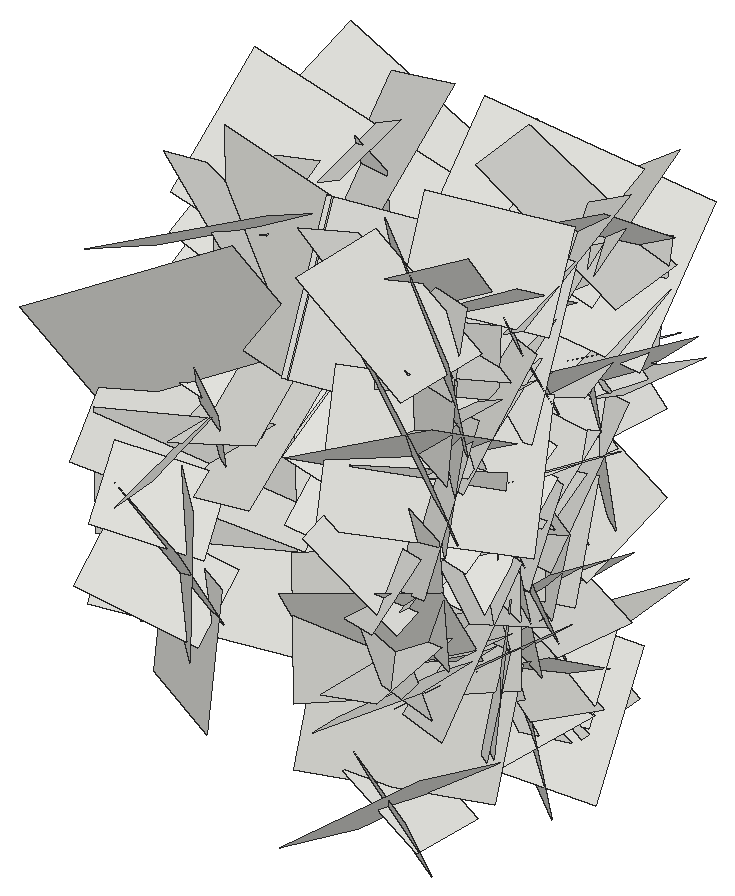
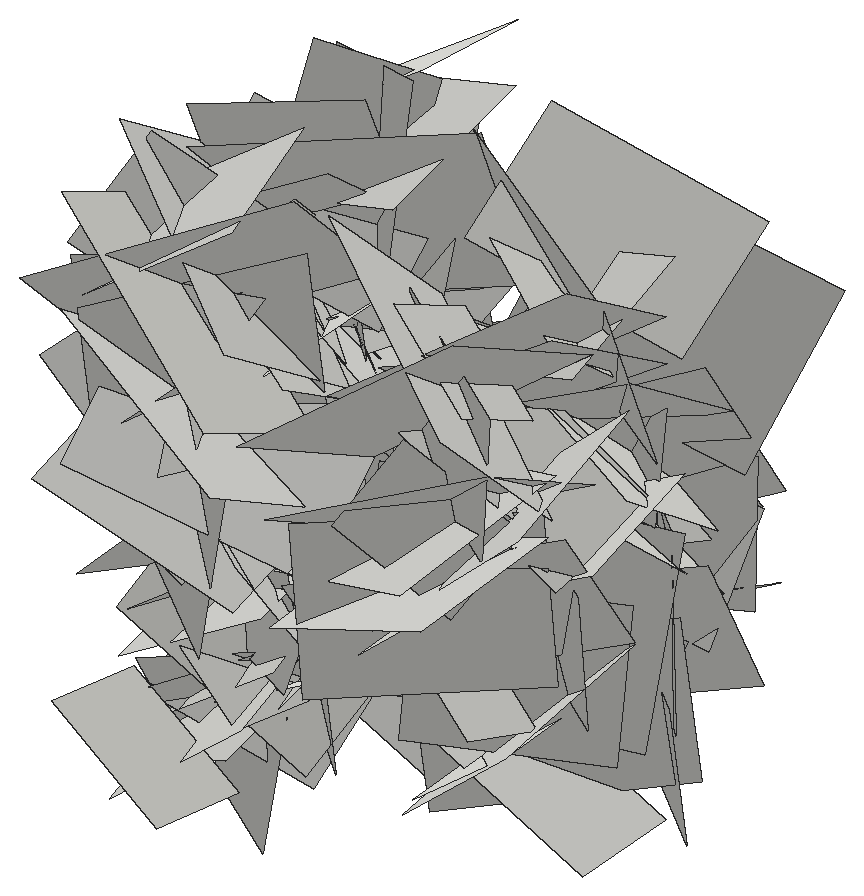
# SketchUp Ruby script. Lengths in inches.
U = 1.inch
M = Sketchup.active_model
def pt(a) = Geom::Point3d.new(a.map { |v| v * U })
def face(e, loops, mat)
  f = e.add_face(loops[0].map { |a| pt(a) })
  loops[1..].each { |l| e.add_face(l.map { |a| pt(a) }).erase! }
  f.material = f.back_material = mat if mat
  f
end
# faces: each face lists its corners as indices into pts; further lists are holes
def faces(e, pts, list, mat = nil) = list.each { |f| face(e, (f[0].is_a?(Array) ? f : [f]).map { |l| l.map { |i| pts[i] } }, mat) }
# xy, xz, yz: faces in a plane at the given z, y or x. An outline is a flat list of corners, or four numbers for a rectangle; further outlines are holes
def ring(l) = l.size == 4 ? [[l[0], l[1]], [l[2], l[1]], [l[2], l[3]], [l[0], l[3]]] : l.each_slice(2).to_a
def flat(e, list, mat, &to3) = list.each { |f| face(e, (f[0].is_a?(Array) ? f : [f]).map { |l| ring(l).map { |u, v| to3.(u, v) } }, mat) }
def xy(e, z, list, mat = nil) = flat(e, list, mat) { |x, y| [x, y, z] }
def xz(e, y, list, mat = nil) = flat(e, list, mat) { |x, z| [x, y, z] }
def yz(e, x, list, mat = nil) = flat(e, list, mat) { |y, z| [x, y, z] }
def lines(e, pts, list) = list.each { |a, b| e.add_line(pt(pts[a]), pt(pts[b])) }
# prism: a flat outline (further loops are holes) pulled along v
def prism(e, loops, v, mat = nil)
  f = face(e, loops, mat); d = Geom::Vector3d.new(v.map { |x| x * U })
  f.pushpull(f.normal.samedirection?(d) ? d.length : -d.length)
end
def box(e, o, s, mat = nil) = prism(e, [[o, [o[0] + s[0], o[1], o[2]], [o[0] + s[0], o[1] + s[1], o[2]], [o[0], o[1] + s[1], o[2]]]], [0, 0, s[2]], mat)
def at(x, y, z, deg = 0) = Geom::Transformation.translation(pt([x, y, z])) * Geom::Transformation.rotation(ORIGIN, Z_AXIS, deg.degrees)
def axes(o, x, y, z) = Geom::Transformation.new([*x, 0, *y, 0, *z, 0, *pt(o).to_a, 1])
def part(name) = M.definitions.add(name)
# library, detail: a bought-in or finely detailed component or shape, given as its bounding box
def library(name, o, s) = part(name).tap { |d| box(d.entities, o, s) }
def detail(e, o, s) = box(e.add_group.entities, o, s)
def put(e, d, t, mat = nil) = e.add_instance(d, t).tap { |i| i.material = mat if mat }
def group(e, t, mat = nil) = e.add_group.tap { |g| g.transformation = t; g.material = mat if mat }.entities
root = M.entities
c1 = part("Component\#6")
p = [[0.01,0,0],[0,3.24,4.54],[4.32,3.24,4.54],[4.33,0,0]]
faces(c1.entities,p,[[0,1,2,3]])
put(root,c1,axes([14.53,185.4,30.76],[-0.02152,-0.00963,-1.2106],[-0.23963,-1.18945,0.01326],[1.26071,-0.22625,-0.01814]))
put(root,c1,axes([14.53,187.18,35.87],[-0.21905,1.32848,-0.23139],[-0.18572,-0.25856,-1.32798],[1.41727,0.17144,-0.20979]))
put(root,c1,axes([18.5,188.41,35.3125],[-0.03073,0.48255,0.4704],[0.10717,0.46862,-0.47449],[-0.70624,0.05011,-0.09248]))
put(root,c1,axes([18.5,183.98,26.9],[0.15473,-0.64925,-0.29626],[-0.07231,-0.3137,0.65387],[-0.75301,-0.10329,-0.12366]))
put(root,c1,axes([18.5,183.4375,30.23],[0.10865,-0.24445,0.66529],[-0.00738,0.67183,0.24793],[-0.75127,-0.04195,0.09378]))
put(root,c1,axes([18.5,185.35,37.93],[0.06077,0.5182,0.40006],[-0.00909,0.40215,-0.51968],[-0.69387,0.04012,0.04185]))
put(root,c1,axes([14.53,182.41,31.86],[-0.21699,-0.67676,1.03332],[0.0082,1.04669,0.68705],[1.3093,-0.11872,0.16695]))
put(root,c1,axes([14.53,181.64,30.57],[0.02444,0.48831,-0.77146],[0.19424,-0.75848,-0.47462],[0.9481,0.1428,0.11713]))
put(root,c1,axes([14.53,184.85,32.98],[-0.15473,1.07562,-0.16592],[0.16403,-0.14519,-1.07739],[1.14193,0.1666,0.13228]))
put(root,c1,axes([18.5,179.78,31.84],[0.01485,0.68647,0.23212],[0.1576,0.2245,-0.67291],[-0.75179,0.06062,-0.13648]))
put(root,c1,axes([18.5,188.93,38.32],[0.06934,0.59373,0.25],[-0.00198,0.25145,-0.59671],[-0.68287,0.05956,0.02711]))
put(root,c1,axes([18.5,193.29,29.97],[-0.02765,-0.60791,0.13872],[0.08921,0.13414,0.60366],[-0.6549,0.04394,0.07638]))
put(root,c1,axes([14.53,189.07,22.99],[0.09993,-0.91741,-0.05408],[0.10319,-0.04408,0.91762],[0.96866,0.09934,-0.09218]))
put(root,c1,axes([14.53,185.63,37.94],[-0.10296,1.07287,0.66666],[-0.13207,0.65722,-1.07584],[1.33238,0.14805,-0.05512]))
put(root,c1,axes([14.53,185.55,26.35],[0.05433,-0.24183,-1.04679],[-0.06418,-1.04696,0.23891],[1.13701,-0.04754,0.0635]))
put(root,c1,axes([18.5,186.02,29.02],[0.12909,0.32312,-0.64935],[0.06195,-0.66067,-0.31779],[-0.76632,0.00102,-0.13508]))
put(root,c1,axes([14.53,190.19,31.82],[0.07854,-1.04848,0.11995],[-0.05802,0.11627,1.05008],[1.11713,0.07975,0.0461]))
put(root,c1,axes([18.5,188.83,29.07],[0.04972,0.59189,0.16701],[0.02122,0.16593,-0.59371],[-0.65156,0.05057,-0.00659]))
put(root,c1,axes([14.53,185.29,39.56],[0.11827,0.82487,-0.51088],[0.03346,-0.51706,-0.82795],[1.02793,-0.07808,0.08573]))
put(root,c1,axes([14.53,186.92,28.87],[0.11772,1.08189,-0.3436],[-0.18933,-0.32428,-1.0788],[1.18826,-0.15885,-0.13785]))
put(root,c1,axes([18.5,191.45,35.51],[0.13227,0.51495,-0.41011],[0.00116,-0.41758,-0.52399],[-0.6978,0.09692,-0.07861]))
put(root,c1,axes([18.5,183.51,30.36],[0.10644,-0.42009,-0.4575],[-0.01901,-0.46521,0.42323],[-0.65811,-0.0545,-0.08622]))
put(root,c1,axes([14.53,184.16,23.6],[0.00632,0.19994,1.20323],[-0.15077,1.19515,-0.1979],[1.28409,0.13934,-0.02916]))
put(root,c1,axes([14.53,189.26,31.29],[0.07003,-0.18149,-1.00879],[0.05402,-1.00905,0.18487],[1.08514,0.06195,0.0559]))
put(root,c1,axes([18.5,191.07,24.72],[0.08022,-0.60182,-0.03468],[0.03515,-0.03074,0.60586],[-0.63802,-0.07736,0.02902]))
put(root,c1,axes([14.53,187.65,25.55],[0.14301,-0.32766,0.90945],[0.11586,0.91755,0.31436],[1.01811,-0.05839,-0.16352]))
put(root,c1,axes([14.53,192.86,38.11],[0.10772,-0.0541,-1.0459],[0.04447,-1.04976,0.05837],[1.10925,0.04734,0.09923]))
put(root,c1,axes([18.5,188.74,27.6],[0.13014,-0.45431,-0.37588],[0.00674,-0.3829,0.46487],[-0.62498,-0.09873,-0.07326]))
put(root,c1,axes([14.53,181.98,27.65],[0.03848,-0.07343,1.06513],[0.13392,1.05855,0.06867],[1.12376,-0.12364,-0.04466]))
put(root,c1,axes([14.53,182.88,33.98],[0.05541,0.90127,0.55592],[0.17138,0.54328,-0.89597],[1.1093,-0.12895,0.11065]))
put(root,c1,axes([14.53,190.1,29],[0.15352,-0.05709,1.12322],[-0.06907,1.13017,0.06585],[1.19015,0.07295,-0.14107]))
put(root,c1,axes([14.53,185.59,36.56],[0.07365,1.00309,0.56692],[0.00038,0.56794,-1.00493],[1.22135,-0.06067,-0.03387]))
put(root,c1,axes([14.53,194.96,38.36],[-0.08597,-0.96025,-0.92678],[-0.03419,-0.92681,0.9631],[1.41421,-0.08078,-0.03305]))
put(root,c1,axes([14.53,188.57,34.3],[-0.02784,1.05016,0.5271],[0.1514,0.52617,-1.0412],[1.23628,-0.04079,0.13938]))
put(root,c1,axes([14.53,186.91,28.91],[-0.08475,0.77289,1.06783],[0.0494,1.07079,-0.77154],[1.39641,0.00903,0.0921]))
put(root,c1,axes([14.53,187.29,32.09],[-0.03087,-0.89426,-0.74249],[0.26998,-0.72958,0.86873],[1.20212,0.14089,-0.21417]))
put(root,c1,axes([14.53,190.5,33.59],[0.11278,1.05886,-0.21225],[0.21462,-0.22906,-1.04119],[1.12442,-0.06248,0.22002]))
put(root,c1,axes([14.53,184.99,36.41],[0.13687,-0.99381,0.45239],[0.15227,0.46704,0.985],[1.14738,0.05657,-0.18469]))
put(root,c1,axes([14.53,181.61,25.33],[-0.14764,0.72138,1.18272],[0.09804,1.19088,-0.71546],[1.46521,-0.007,0.16705]))
put(root,c1,axes([14.53,187.26,33.24],[0.066,-0.95024,-0.64083],[0.19237,-0.6255,0.94515],[1.19957,0.15259,-0.11631]))
put(root,c1,axes([14.53,188.72,38.18],[0.108,1.17484,0.54266],[-0.09899,0.5496,-1.17232],[1.36819,-0.05298,-0.12766]))
put(root,c1,axes([14.53,180.73,30.67],[0.05707,0.69485,1.12415],[-0.04583,1.1254,-0.69356],[1.4001,0.00851,-0.06852]))
put(root,c1,axes([14.53,188.1875,39.24],[0.00053,-0.50504,-1.25708],[0.1621,-1.24903,0.50186],[1.42684,0.14209,-0.05655]))
put(root,c1,axes([14.53,186.51,25.44],[-0.00901,-0.3677,1.34811],[0.26845,1.32541,0.3631],[1.45667,-0.24653,-0.05858]))
put(root,c1,axes([14.53,190.14,35.27],[0.30668,1.10496,-0.445],[0.14325,-0.48543,-1.11748],[1.25452,-0.21469,0.23639]))
put(root,c1,axes([28.31,190.14,35.27],[-0.30668,1.10496,-0.445],[-0.14325,-0.48543,-1.11748],[-1.25452,-0.21469,0.23639]))
put(root,c1,axes([28.31,186.51,25.44],[0.00901,-0.3677,1.34811],[-0.26845,1.32541,0.3631],[-1.45667,-0.24653,-0.05858]))
put(root,c1,axes([28.31,188.1875,39.24],[-0.00053,-0.50504,-1.25708],[-0.1621,-1.24903,0.50186],[-1.42684,0.14209,-0.05655]))
put(root,c1,axes([28.31,180.73,30.67],[-0.05707,0.69485,1.12415],[0.04583,1.1254,-0.69356],[-1.4001,0.00851,-0.06852]))
put(root,c1,axes([28.31,188.72,38.18],[-0.108,1.17484,0.54266],[0.09899,0.5496,-1.17232],[-1.36819,-0.05298,-0.12766]))
put(root,c1,axes([28.31,187.26,33.24],[-0.066,-0.95024,-0.64083],[-0.19237,-0.6255,0.94515],[-1.19957,0.15259,-0.11631]))
put(root,c1,axes([28.31,181.61,25.33],[0.14764,0.72138,1.18272],[-0.09804,1.19088,-0.71546],[-1.46521,-0.007,0.16705]))
put(root,c1,axes([28.31,184.99,36.41],[-0.13687,-0.99381,0.45239],[-0.15227,0.46704,0.985],[-1.14738,0.05657,-0.18469]))
put(root,c1,axes([28.31,190.5,33.59],[-0.11278,1.05886,-0.21225],[-0.21462,-0.22906,-1.04119],[-1.12442,-0.06248,0.22002]))
put(root,c1,axes([28.31,187.29,32.09],[0.03087,-0.89426,-0.74249],[-0.26998,-0.72958,0.86873],[-1.20212,0.14089,-0.21417]))
put(root,c1,axes([28.31,186.91,28.91],[0.08475,0.77289,1.06783],[-0.0494,1.07079,-0.77154],[-1.39641,0.00903,0.0921]))
put(root,c1,axes([28.31,188.57,34.3],[0.02784,1.05016,0.5271],[-0.1514,0.52617,-1.0412],[-1.23628,-0.04079,0.13938]))
put(root,c1,axes([28.31,194.96,38.36],[0.08597,-0.96025,-0.92678],[0.03419,-0.92681,0.9631],[-1.41421,-0.08078,-0.03305]))
put(root,c1,axes([28.31,185.59,36.56],[-0.07365,1.00309,0.56692],[-0.00038,0.56794,-1.00493],[-1.22135,-0.06067,-0.03387]))
put(root,c1,axes([28.31,190.1,29],[-0.15352,-0.05709,1.12322],[0.06907,1.13017,0.06585],[-1.19015,0.07295,-0.14107]))
put(root,c1,axes([28.31,182.88,33.98],[-0.05541,0.90127,0.55592],[-0.17138,0.54328,-0.89597],[-1.1093,-0.12895,0.11065]))
put(root,c1,axes([28.31,181.98,27.65],[-0.03848,-0.07343,1.06513],[-0.13392,1.05855,0.06867],[-1.12376,-0.12364,-0.04466]))
put(root,c1,axes([24.34,188.74,27.6],[-0.13014,-0.45431,-0.37588],[-0.00674,-0.3829,0.46487],[0.62498,-0.09873,-0.07326]))
put(root,c1,axes([28.31,192.86,38.11],[-0.10772,-0.0541,-1.0459],[-0.04447,-1.04976,0.05837],[-1.10925,0.04734,0.09923]))
put(root,c1,axes([28.31,187.65,25.55],[-0.14301,-0.32766,0.90945],[-0.11586,0.91755,0.31436],[-1.01811,-0.05839,-0.16352]))
put(root,c1,axes([24.34,191.07,24.72],[-0.08022,-0.60182,-0.03468],[-0.03515,-0.03074,0.60586],[0.63802,-0.07736,0.02902]))
put(root,c1,axes([28.31,189.26,31.29],[-0.07003,-0.18149,-1.00879],[-0.05402,-1.00905,0.18487],[-1.08514,0.06195,0.0559]))
put(root,c1,axes([28.31,184.16,23.6],[-0.00632,0.19994,1.20323],[0.15077,1.19515,-0.1979],[-1.28409,0.13934,-0.02916]))
put(root,c1,axes([24.34,183.51,30.36],[-0.10644,-0.42009,-0.4575],[0.01901,-0.46521,0.42323],[0.65811,-0.0545,-0.08622]))
put(root,c1,axes([24.34,191.45,35.51],[-0.13227,0.51495,-0.41011],[-0.00116,-0.41758,-0.52399],[0.6978,0.09692,-0.07861]))
put(root,c1,axes([28.31,186.92,28.87],[-0.11772,1.08189,-0.3436],[0.18933,-0.32428,-1.0788],[-1.18826,-0.15885,-0.13785]))
put(root,c1,axes([28.31,185.29,39.56],[-0.11827,0.82487,-0.51088],[-0.03346,-0.51706,-0.82795],[-1.02793,-0.07808,0.08573]))
put(root,c1,axes([24.34,188.83,29.07],[-0.04972,0.59189,0.16701],[-0.02122,0.16593,-0.59371],[0.65156,0.05057,-0.00659]))
put(root,c1,axes([28.31,190.19,31.82],[-0.07854,-1.04848,0.11995],[0.05802,0.11627,1.05008],[-1.11713,0.07975,0.0461]))
put(root,c1,axes([24.34,186.02,29.02],[-0.12909,0.32312,-0.64935],[-0.06195,-0.66067,-0.31779],[0.76632,0.00102,-0.13508]))
put(root,c1,axes([28.31,185.55,26.35],[-0.05433,-0.24183,-1.04679],[0.06418,-1.04696,0.23891],[-1.13701,-0.04754,0.0635]))
put(root,c1,axes([28.31,185.63,37.94],[0.10296,1.07287,0.66666],[0.13207,0.65722,-1.07584],[-1.33238,0.14805,-0.05512]))
put(root,c1,axes([28.31,189.07,22.99],[-0.09993,-0.91741,-0.05408],[-0.10319,-0.04408,0.91762],[-0.96866,0.09934,-0.09218]))
put(root,c1,axes([24.34,193.29,29.97],[0.02765,-0.60791,0.13872],[-0.08921,0.13414,0.60366],[0.6549,0.04394,0.07638]))
put(root,c1,axes([24.34,188.93,38.32],[-0.06934,0.59373,0.25],[0.00198,0.25145,-0.59671],[0.68287,0.05956,0.02711]))
put(root,c1,axes([24.34,179.78,31.84],[-0.01485,0.68647,0.23212],[-0.1576,0.2245,-0.67291],[0.75179,0.06062,-0.13648]))
put(root,c1,axes([28.31,184.85,32.98],[0.15473,1.07562,-0.16592],[-0.16403,-0.14519,-1.07739],[-1.14193,0.1666,0.13228]))
put(root,c1,axes([28.31,181.64,30.57],[-0.02444,0.48831,-0.77146],[-0.19424,-0.75848,-0.47462],[-0.9481,0.1428,0.11713]))
put(root,c1,axes([28.31,182.41,31.86],[0.21699,-0.67676,1.03332],[-0.0082,1.04669,0.68705],[-1.3093,-0.11872,0.16695]))
put(root,c1,axes([24.34,185.35,37.93],[-0.06077,0.5182,0.40006],[0.00909,0.40215,-0.51968],[0.69387,0.04012,0.04185]))
put(root,c1,axes([24.34,183.4375,30.23],[-0.10865,-0.24445,0.66529],[0.00738,0.67183,0.24793],[0.75127,-0.04195,0.09378]))
put(root,c1,axes([24.34,183.98,26.9],[-0.15473,-0.64925,-0.29626],[0.07231,-0.3137,0.65387],[0.75301,-0.10329,-0.12366]))
put(root,c1,axes([24.34,188.41,35.3125],[0.03073,0.48255,0.4704],[-0.10717,0.46862,-0.47449],[0.70624,0.05011,-0.09248]))
put(root,c1,axes([28.31,187.18,35.87],[0.21905,1.32848,-0.23139],[0.18572,-0.25856,-1.32798],[-1.41727,0.17144,-0.20979]))
put(root,c1,axes([28.31,185.4,30.76],[0.02152,-0.00963,-1.2106],[0.23963,-1.18945,0.01326],[-1.26071,-0.22625,-0.01814]))
put(root,c1,axes([24.34,183.74,37.84],[0.08456,-0.37494,0.46177],[-0.03825,0.46199,0.38136],[0.62935,0.07846,-0.03886]))
put(root,c1,axes([24.34,188.62,32.29],[-0.0866,-0.74743,0.19758],[-0.06186,0.20408,0.74787],[0.81715,-0.06376,0.07755]))
put(root,c1,axes([24.34,184.65,28.76],[0.04824,-0.62434,-0.28052],[-0.09786,-0.28417,0.61748],[0.7189,0.00321,0.10288]))
put(root,c1,axes([28.31,186.48,30.64],[-0.03295,0.70699,0.47041],[-0.18441,0.45544,-0.69599],[-0.88105,-0.12176,0.12808]))
put(root,c1,axes([28.31,180.55,24.45],[-0.04702,0.95483,-0.28451],[0.08229,-0.28062,-0.95386],[-1.05288,-0.06457,-0.06184]))
put(root,c1,axes([28.31,184.8,33.37],[-0.19651,0.19461,-0.78555],[0.01158,-0.80522,-0.20206],[-0.85778,-0.05545,0.17724]))
put(root,c1,axes([28.31,181.12,36.49],[0.0887,0.85058,-0.45713],[-0.14057,-0.44437,-0.85112],[-1.01388,0.13603,0.07801]))
put(root,c1,axes([24.34,182.11,23.57],[-0.01533,0.32032,-0.55846],[0.07998,-0.55391,-0.31966],[0.67773,0.07262,0.02509]))
put(root,c1,axes([24.34,186.27,36.66],[-0.23271,0.08267,-1.0169],[-0.17131,-1.02986,-0.04883],[1.06781,-0.14721,-0.22945]))
put(root,c1,axes([24.34,181.88,29.24],[0.0732,0.47057,-0.46808],[-0.06498,-0.46407,-0.47558],[0.70054,-0.09222,0.00479]))
put(root,c1,axes([24.34,188.01,25.87],[-0.18323,0.88768,-0.1275],[-0.06793,-0.14175,-0.89995],[0.94816,0.16139,-0.08912]))
put(root,c1,axes([28.31,186.85,26],[-0.04759,0.74401,-0.43208],[-0.09551,-0.43435,-0.73856],[-0.90698,0.0067,0.10045]))
put(root,c1,axes([28.31,182.62,33.52],[0.16113,0.63843,0.91206],[0.00988,0.91976,-0.64538],[-1.18006,0.09488,0.11913]))
put(root,c1,axes([24.34,188.3,31.13],[-0.1103,-0.11339,-0.88165],[-0.13763,-0.87621,0.12802],[0.93214,-0.14279,-0.08543]))
put(root,c1,axes([28.31,182.86,27.86],[-0.00866,0.87216,-0.09866],[-0.12421,-0.09886,-0.86427],[-0.92206,0.00513,0.11735]))
put(root,c1,axes([24.34,188.48,31.6],[0.00806,0.51701,-0.38199],[0.06142,-0.38101,-0.51453],[0.67861,0.02834,0.0511]))
put(root,c1,axes([24.34,189.49,31],[-0.19159,0.03614,-0.77666],[0.1449,-0.78347,-0.06827],[0.81131,0.14846,-0.17121]))
put(root,c1,axes([28.31,186.8,27.07],[0.11611,-1.02809,0.5245],[0.14127,0.5346,1.02006],[-1.21522,-0.03608,0.16869]))
put(root,c1,axes([24.34,181.75,22.9],[0.07496,0.59984,0.04506],[0.05269,0.03939,-0.60235],[0.63545,-0.07402,0.04463]))
put(root,c1,axes([28.31,190.89,25.45],[0.07637,-0.93381,0.1535],[-0.06656,0.14888,0.93522],[-1.00091,-0.08115,-0.05048]))
put(root,c1,axes([28.31,189.24,21.76],[-0.15995,-0.688,0.38857],[0.02017,0.39231,0.70202],[-0.83731,0.14088,-0.05731]))
put(root,c1,axes([24.34,186.9,33.68],[-0.12726,-0.80704,-0.07778],[0.05104,-0.08559,0.81372],[0.85791,-0.11462,-0.05995]))
put(root,c1,axes([24.34,183.3,35.54],[0.06853,-0.0517,0.64839],[0.02911,0.65122,0.04919],[0.68886,-0.02238,-0.06659]))
put(root,c1,axes([28.31,182.91,34.72],[0.14912,-0.41506,0.98502],[0.044,0.99488,0.41329],[-1.13217,-0.016,0.1458]))
put(root,c1,axes([28.31,191.48,24.4],[0.24044,-0.84726,-0.84182],[0.11443,-0.83882,0.87332],[-1.26085,-0.2377,-0.08127]))
put(root,c1,axes([24.34,194.3125,23.26],[-0.02367,-0.75059,-0.08188],[0.02978,-0.08269,0.75031],[0.79979,-0.01914,-0.03036]))
put(root,c1,axes([28.31,189.58,22.99],[0.08755,-0.94666,0.34405],[0.04779,0.34833,0.94763],[-1.06661,-0.0621,0.0707]))
put(root,c1,axes([28.31,183.5625,38.07],[-0.03427,-0.86867,-0.02883],[0.01016,-0.0292,0.8692],[-0.92124,0.03199,0.01066]))
put(root,c1,axes([24.34,186.98,23.44],[-0.07046,0.41434,0.63319],[0.10971,0.63463,-0.40442],[0.79457,-0.05088,0.11199]))
put(root,c1,axes([28.31,186.99,20.26],[-0.04681,-0.17583,0.86867],[0.05724,0.86759,0.17835],[-0.93771,0.06173,-0.03248]))
put(root,c1,axes([24.34,182.78,23.92],[-0.06221,-0.24398,0.83625],[-0.07047,0.83695,0.23952],[0.92069,0.04758,0.07484]))
put(root,c1,axes([28.31,187.32,34.27],[-0.05201,-0.4187,0.7383],[0.02779,0.73844,0.42051],[-0.89926,0.04704,-0.0297]))
put(root,c1,axes([24.34,187.84,31.26],[0.01205,0.8882,0.30464],[-0.22592,0.29915,-0.86424],[0.96935,0.05868,-0.20521]))
put(root,c1,axes([24.34,187.61,26.86],[-0.07932,-0.16974,-0.83453],[-0.0041,-0.83766,0.17072],[0.9027,-0.01872,-0.07255]))
put(root,c1,axes([24.34,184.84,39.1],[0.02023,-0.20369,-0.6632],[0.11732,-0.65406,0.20407],[0.72599,0.11137,-0.0145]))
put(root,c1,axes([28.31,180.54,27.52],[-0.00647,0.86334,-0.00303],[0.00368,-0.003,-0.86336],[-0.91514,-0.00612,-0.00345]))
put(root,c1,axes([28.31,189.53,40.3125],[0.07096,0.70634,-0.4758],[-0.12627,-0.46481,-0.70678],[-0.89387,0.12173,0.06207]))
put(root,c1,axes([28.31,192.58,32.17],[-0.11188,-0.86522,-0.03173],[0.14554,-0.04829,0.85998],[-0.90613,0.09907,0.14204]))
put(root,c1,axes([28.31,185.86,28.71],[0.06844,0.29244,0.76285],[-0.17475,0.75415,-0.27515],[-0.84819,-0.13178,0.11824]))
put(root,c1,axes([24.34,188.23,41.22],[-0.26749,1.02168,-0.17372],[0.00845,-0.17688,-1.05183],[1.0985,0.25014,-0.03421]))
put(root,c1,axes([28.31,187.08,35.11],[0.23629,-0.52338,-1.02054],[0.13084,-1.02265,0.55142],[-1.20867,-0.21302,-0.13982]))
put(root,c1,axes([24.34,187.74,23.43],[-0.08523,-0.9506,0.05636],[-0.09187,0.06363,0.94959],[1.00521,-0.07479,0.09156]))
put(root,c1,axes([24.34,184.52,38.07],[-0.06477,0.36641,0.7198],[0.11209,0.71927,-0.35717],[0.84878,-0.06703,0.10209]))
put(root,c1,axes([24.34,184.92,37.05],[0.01613,-0.13323,-0.78421],[0.01491,-0.78419,0.1335],[0.84304,0.01642,0.01265]))
